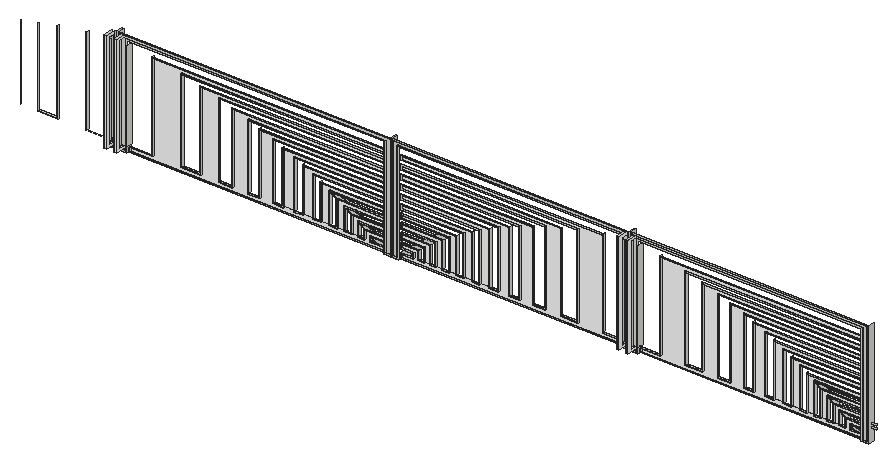
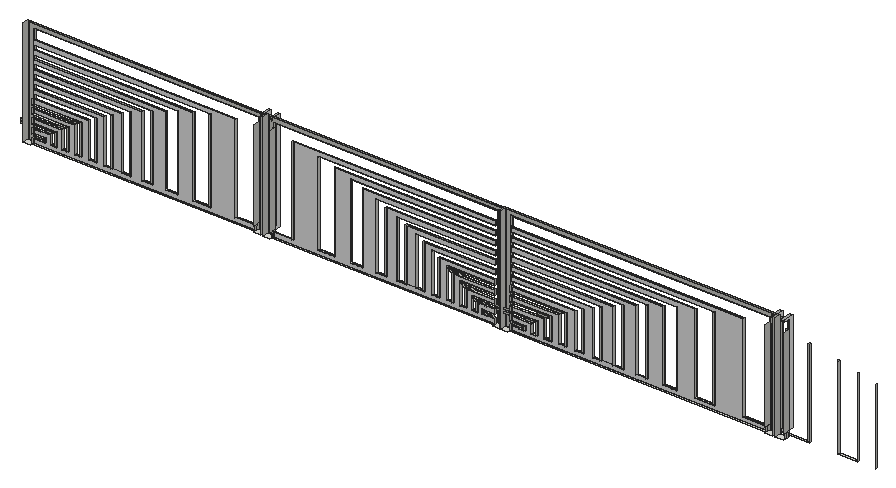
# SketchUp Ruby script. Lengths in inches.
U = 1.inch
M = Sketchup.active_model
def pt(a) = Geom::Point3d.new(a.map { |v| v * U })
def face(e, loops, mat)
  f = e.add_face(loops[0].map { |a| pt(a) })
  loops[1..].each { |l| e.add_face(l.map { |a| pt(a) }).erase! }
  f.material = f.back_material = mat if mat
  f
end
# faces: each face lists its corners as indices into pts; further lists are holes
def faces(e, pts, list, mat = nil) = list.each { |f| face(e, (f[0].is_a?(Array) ? f : [f]).map { |l| l.map { |i| pts[i] } }, mat) }
# xy, xz, yz: faces in a plane at the given z, y or x. An outline is a flat list of corners, or four numbers for a rectangle; further outlines are holes
def ring(l) = l.size == 4 ? [[l[0], l[1]], [l[2], l[1]], [l[2], l[3]], [l[0], l[3]]] : l.each_slice(2).to_a
def flat(e, list, mat, &to3) = list.each { |f| face(e, (f[0].is_a?(Array) ? f : [f]).map { |l| ring(l).map { |u, v| to3.(u, v) } }, mat) }
def xy(e, z, list, mat = nil) = flat(e, list, mat) { |x, y| [x, y, z] }
def xz(e, y, list, mat = nil) = flat(e, list, mat) { |x, z| [x, y, z] }
def yz(e, x, list, mat = nil) = flat(e, list, mat) { |y, z| [x, y, z] }
def lines(e, pts, list) = list.each { |a, b| e.add_line(pt(pts[a]), pt(pts[b])) }
# prism: a flat outline (further loops are holes) pulled along v
def prism(e, loops, v, mat = nil)
  f = face(e, loops, mat); d = Geom::Vector3d.new(v.map { |x| x * U })
  f.pushpull(f.normal.samedirection?(d) ? d.length : -d.length)
end
def box(e, o, s, mat = nil) = prism(e, [[o, [o[0] + s[0], o[1], o[2]], [o[0] + s[0], o[1] + s[1], o[2]], [o[0], o[1] + s[1], o[2]]]], [0, 0, s[2]], mat)
def at(x, y, z, deg = 0) = Geom::Transformation.translation(pt([x, y, z])) * Geom::Transformation.rotation(ORIGIN, Z_AXIS, deg.degrees)
def axes(o, x, y, z) = Geom::Transformation.new([*x, 0, *y, 0, *z, 0, *pt(o).to_a, 1])
def part(name) = M.definitions.add(name)
# library, detail: a bought-in or finely detailed component or shape, given as its bounding box
def library(name, o, s) = part(name).tap { |d| box(d.entities, o, s) }
def detail(e, o, s) = box(e.add_group.entities, o, s)
def put(e, d, t, mat = nil) = e.add_instance(d, t).tap { |i| i.material = mat if mat }
def group(e, t, mat = nil) = e.add_group.tap { |g| g.transformation = t; g.material = mat if mat }.entities
root = M.entities
M.materials.add("[Color_000]").color = [255, 255, 255]
xy(root,0,[[821.45,11.31,827.35,15.56],[828.58,11.31,834.47,15.56],[1013.27,11.31,1019.16,15.56],[1018.58,11.31,1023.71,15.56],[1179.26,11.31,1184.39,15.56],
  [1185.46,11.31,1190.59,15.56],[1346.14,11.31,1351.27,15.56],[834.47,12.93,1013.27,14.31],[1023.71,12.93,1179.26,14.31],[1190.59,12.93,1346.14,14.31]])
xy(root,0.49,[[835.26,12.93,1012.48,13.56],[1024.39,12.93,1178.58,13.56],[1191.27,12.93,1345.46,13.56]])
xy(root,0.7,[[822.57,11.31,826.23,11.81],[829.7,11.31,833.35,11.81],[1014.39,11.31,1018.04,11.81],[1019.55,11.31,1022.73,11.81],[1180.23,11.31,1183.41,11.81],
  [1186.43,11.31,1189.61,11.81],[1347.11,11.31,1350.3,11.81]])
xy(root,2.12,[[823.54,4.75,825.37,11.81],[830.56,4.75,832.38,11.81],[1181.08,4.75,1182.66,11.81],[1187.18,4.75,1188.77,11.81]],"[Color_000]")
xy(root,3.2,[[771.16,12.93,785.19,13.56],[804.64,12.93,820.67,13.56],[835.26,12.93,851.28,13.56],[870.74,12.93,884.76,13.56],[897.07,12.93,907.12,13.56],
  [917.52,12.93,926.1,13.56],[934.55,12.93,942.21,13.56],[949.3125,12.93,956.23,13.56],[962.35,12.93,968.64,13.56],[974.05,12.93,979.79,13.56],
  [984.5625,12.93,989.91,13.56],[993.96,12.93,999.18,13.56],[1002.58,12.93,1006.64,13.56],[1006.64,12.93,1012.48,13.56],[1024.39,12.93,1029.48,13.56],
  [1029.48,12.93,1033,13.56],[1035.96,12.93,1040.51,13.56],[1044.03,12.93,1048.68,13.56],[1052.83,12.93,1057.83,13.56],[1062.53,12.93,1068,13.56],
  [1073.33,12.93,1079.35,13.56],[1085.53,12.93,1092.19,13.56],[1099.55,12.93,1107,13.56],[1116.06,12.93,1124.8,13.56],[1135.51,12.93,1147.71,13.56],
  [1164.63,12.93,1178.58,13.56],[1191.27,12.93,1205.21,13.56],[1222.14,12.93,1234.34,13.56],[1245.05,12.93,1253.79,13.56],[1262.84,12.93,1270.3,13.56],
  [1277.65,12.93,1284.32,13.56],[1290.5,12.93,1296.52,13.56],[1301.84,12.93,1307.3125,13.56],[1312.02,12.93,1317.01,13.56],[1321.17,12.93,1325.82,13.56],
  [1329.34,12.93,1333.88,13.56],[1336.84,12.93,1340.37,13.56],[1340.37,12.93,1345.46,13.56]])
xy(root,3.52,[[823.54,7.12,825.37,11.81],[830.56,7.12,832.38,11.81],[1181.08,7.12,1182.66,11.81],[1187.18,7.12,1188.77,11.81]],"[Color_000]")
xy(root,3.7,[[771.95,12.93,784.4,12.93,784.4,14.31,771.95,14.17],[871.53,12.93,871.53,14.31,883.97,14.17,883.97,12.93],[897.86,12.93,897.86,14.02,906.33,13.93,906.33,12.93],[918.3125,12.93,918.3125,13.8,925.31,13.73,925.31,12.93],[935.33,12.93,935.33,13.62,941.43,13.55,941.43,12.93],
  [950.1,12.93,950.1,13.46,955.44,13.4,955.44,12.93],[963.14,12.93,963.14,13.32,967.85,13.27,967.85,12.93],[974.83,12.93,974.83,13.19,979,13.15,979,12.93],[985.35,12.93,985.35,13.08,989.12,13.04,989.12,12.93],[994.75,12.93,994.75,12.97,998.39,12.93],
  [998.39,12.93,994.75,12.97,994.75,14.31,998.39,14.31],[1003.37,12.93,1006.64,14.31],[1029.48,12.93,1032.32,14.31],[1036.65,12.93,1039.82,12.93,1039.82,12.97],[1036.65,12.93,1039.82,12.97,1039.82,14.31,1036.65,14.31],
  [1044.71,12.93,1047.99,12.93,1047.99,13.08,1044.71,13.04],[1053.52,12.93,1057.15,12.93,1057.15,13.19,1053.52,13.15],[1063.22,12.93,1067.32,12.93,1067.32,13.32,1063.22,13.27],[1074.02,12.93,1078.67,12.93,1078.67,13.46,1074.02,13.4],[1086.21,12.93,1091.51,12.93,1091.51,13.62,1086.21,13.55],
  [1100.23,12.93,1106.32,12.93,1106.32,13.8,1100.23,13.73],[1116.74,12.93,1124.11,12.93,1124.11,14.02,1116.74,13.93],[1136.19,12.93,1147.02,12.93,1147.02,14.31,1136.19,14.17],[1222.82,12.93,1222.82,14.31,1233.65,14.17,1233.65,12.93],[1245.73,12.93,1245.73,14.02,1253.1,13.93,1253.1,12.93],
  [1263.53,12.93,1263.53,13.8,1269.61,13.73,1269.61,12.93],[1278.34,12.93,1278.34,13.62,1283.64,13.55,1283.64,12.93],[1291.18,12.93,1291.18,13.46,1295.83,13.4,1295.83,12.93],[1302.53,12.93,1302.53,13.32,1306.63,13.27,1306.63,12.93],[1312.7,12.93,1312.7,13.19,1316.33,13.15,1316.33,12.93],
  [1321.85,12.93,1321.85,13.08,1325.13,13.04,1325.13,12.93],[1330.03,12.93,1330.03,12.97,1333.2,12.93],[1333.2,12.93,1330.03,12.97,1330.03,14.31,1333.2,14.31],[1337.53,12.93,1340.37,14.31]])
xy(root,6.12,[[1003.37,12.93,1010.01,14.31],[1026.55,12.93,1032.32,14.31],[1337.53,12.93,1343.3,14.31]])
xy(root,6.62,[[1002.58,12.93,1010.01,13.56],[1010.01,12.93,1012.48,13.56],[1024.39,12.93,1026.55,13.56],[1026.55,12.93,1033,13.56],[1336.84,12.93,1343.3,13.56],
  [1343.3,12.93,1345.46,13.56]])
xy(root,9.32,[[999.18,12.93,1005.03,13.56],[1005.03,12.93,1006.64,13.56],[1006.64,12.93,1012.48,13.56],[1024.39,12.93,1029.48,13.56],[1029.48,12.93,1030.875,13.56],
  [1030.875,12.93,1035.96,13.56],[1333.88,12.93,1338.97,13.56],[1338.97,12.93,1340.37,13.56],[1340.37,12.93,1345.46,13.56]])
xy(root,9.82,[[998.39,12.93,1005.03,14.31],[1005.03,12.93,1006.64,14.31],[1006.64,12.93,1013.27,14.31],[1023.71,12.93,1029.48,14.31],[1029.48,12.93,1030.875,14.31],
  [1030.875,12.93,1036.65,14.31],[1333.2,12.93,1338.97,14.31],[1338.97,12.93,1340.37,14.31],[1340.37,12.93,1346.14,14.31]])
xy(root,12.24,[[994.75,12.93,1001.75,14.31],[1001.75,12.93,1013.27,14.31],[1023.71,12.93,1033.73,14.31],[1033.73,12.93,1039.82,14.31],[1330.03,12.93,1336.12,14.31],
  [1336.12,12.93,1346.14,14.31]])
xy(root,12.74,[[993.96,12.93,1001.75,13.56],[1001.75,12.93,1012.48,13.56],[1024.39,12.93,1033.73,13.56],[1033.73,12.93,1040.51,13.56],[1329.34,12.93,1336.12,13.56],
  [1336.12,12.93,1345.46,13.56]])
xy(root,15.44,[[989.91,12.93,996.13,13.56],[996.13,12.93,1012.48,13.56],[1024.39,12.93,1038.62,13.56],[1038.62,12.93,1044.03,13.56],[1325.82,12.93,1331.23,13.56],
  [1331.23,12.93,1345.46,13.56]])
xy(root,15.9375,[[989.12,12.93,996.13,14.31],[996.13,12.93,1013.27,14.31],[1023.71,12.93,1038.62,14.31],[1038.62,12.93,1044.71,14.31],[1325.13,12.93,1331.23,14.31],
  [1331.23,12.93,1346.14,14.31]])
xy(root,18.36,[[985.35,12.93,992.44,14.31],[992.44,12.93,1013.27,14.31],[1023.71,12.93,1041.83,14.31],[1041.83,12.93,1047.99,14.31],[1321.85,12.93,1328.02,14.31],
  [1328.02,12.93,1346.14,14.31]])
xy(root,18.86,[[984.5625,12.93,992.44,13.56],[992.44,12.93,1012.48,13.56],[1024.39,12.93,1041.83,13.56],[1041.83,12.93,1048.68,13.56],[1321.17,12.93,1328.02,13.56],
  [1328.02,12.93,1345.46,13.56]])
xy(root,21.57,[[979.79,12.93,986.45,13.56],[986.45,12.93,1012.48,13.56],[1024.39,12.93,1047.04,13.56],[1047.04,12.93,1052.83,13.56],[1317.01,12.93,1322.8125,13.56],
  [1322.8125,12.93,1345.46,13.56]])
xy(root,22.06,[[979,12.93,986.45,14.31],[986.45,12.93,1013.27,14.31],[1023.71,12.93,1047.04,14.31],[1047.04,12.93,1053.52,14.31],[1316.33,12.93,1322.8125,14.31],
  [1322.8125,12.93,1346.14,14.31]])
xy(root,24.48,[[974.83,12.93,982.29,14.31],[982.29,12.93,1013.27,14.31],[1023.71,12.93,1050.66,14.31],[1050.66,12.93,1057.15,14.31],[1312.7,12.93,1319.1875,14.31],
  [1319.1875,12.93,1346.14,14.31]])
xy(root,24.98,[[974.05,12.93,982.29,13.56],[982.29,12.93,1012.48,13.56],[1024.39,12.93,1050.66,13.56],[1050.66,12.93,1057.83,13.56],[1312.02,12.93,1319.1875,13.56],
  [1319.1875,12.93,1345.46,13.56]])
xz(root,4.75,[[823.54,2.12,825.37,72.7],[830.56,2.12,832.38,72.7],[1181.08,2.12,1182.66,72.7],[1187.18,2.12,1188.77,72.7]],"[Color_000]")
xz(root,7.12,[[823.54,3.52,825.37,71.3],[830.56,3.52,832.38,71.3],[1181.08,3.52,1182.66,71.3],[1187.18,3.52,1188.77,71.3]],"[Color_000]")
xz(root,11.31,[[[828.58,0,828.58,73.9,1019.16,73.9,1019.16,0,1013.27,0,1013.27,70.2,834.47,70.2,834.47,0],[829.7,0.7,833.35,0.7,833.35,70.9,1014.39,70.9,1014.39,0.7,1018.04,0.7,1018.04,73.2,829.7,73.2]],[[1018.58,0,1023.71,0,1023.71,70.2,1179.26,70.2,1179.26,0,1184.39,0,1184.39,73.9,1018.58,73.9],[1019.55,0.7,1019.55,73.2,1183.41,73.2,1183.41,0.7,1180.23,0.7,1180.23,70.9,1022.73,70.9,1022.73,0.7]],[[1185.46,0,1185.46,73.9,1351.27,73.9,1351.27,0,1346.14,0,1346.14,70.2,1190.59,70.2,1190.59,0],[1186.43,0.7,1189.61,0.7,1189.61,70.9,1347.11,70.9,1347.11,0.7,1350.3,0.7,1350.3,73.2,1186.43,73.2]]])
xz(root,11.81,[[[829.7,0.7,829.7,73.2,1018.04,73.2,1018.04,0.7,1014.39,0.7,1014.39,70.9,833.35,70.9,833.35,0.7],[830.56,71.3,832.38,72.7],[830.56,2.12,832.38,3.52]],[[1019.55,0.7,1022.73,0.7,1022.73,70.9,1180.23,70.9,1180.23,0.7,1183.41,0.7,1183.41,73.2,1019.55,73.2],[1181.08,71.3,1182.66,72.7],[1181.08,2.12,1182.66,3.52]],[[1186.43,0.7,1186.43,73.2,1350.3,73.2,1350.3,0.7,1347.11,0.7,1347.11,70.9,1189.61,70.9,1189.61,0.7],[1187.18,71.3,1188.77,72.7],[1187.18,2.12,1188.77,3.52]]])
xz(root,12.93,[[[834.47,0,834.47,3.7,850.5,3.7,850.5,64.91,1013.27,64.91,1013.27,61.21,871.53,61.21,871.53,3.7,883.97,3.7,883.97,58.79,1013.27,58.79,1013.27,55.09,897.86,55.09,897.86,3.7,906.33,3.7,906.33,52.67,1013.27,52.67,1013.27,48.97,918.3125,48.97,918.3125,3.7,925.31,3.7,925.31,46.54,1013.27,46.54,1013.27,42.85,935.33,42.85,935.33,3.7,941.43,3.7,941.43,40.42,1013.27,40.42,1013.27,36.73,950.1,36.73,950.1,3.7,955.44,3.7,955.44,34.3,1013.27,34.3,1013.27,30.61,963.14,30.61,963.14,3.7,967.85,3.7,967.85,28.18,1013.27,28.18,1013.27,24.48,974.83,24.48,974.83,3.7,979,3.7,979,22.06,1013.27,22.06,1013.27,18.36,985.35,18.36,985.35,3.7,989.12,3.7,989.12,15.9375,1013.27,15.9375,1013.27,12.24,994.75,12.24,994.75,3.7,998.39,3.7,998.39,9.82,1013.27,9.82,1013.27,6.12,1003.37,6.12,1003.37,3.7,1013.27,3.7,1013.27,0],[835.26,0.49,1012.48,0.49,1012.48,3.2,1002.58,3.2,1002.58,6.62,1012.48,6.62,1012.48,9.32,999.18,9.32,999.18,3.2,993.96,3.2,993.96,12.74,1012.48,12.74,1012.48,15.44,989.91,15.44,989.91,3.2,984.5625,3.2,984.5625,18.86,1012.48,18.86,1012.48,21.57,979.79,21.57,979.79,3.2,974.05,3.2,974.05,24.98,1012.48,24.98,1012.48,27.6875,968.64,27.6875,968.64,3.2,962.35,3.2,962.35,31.1,1012.48,31.1,1012.48,33.81,956.23,33.81,956.23,3.2,949.3125,3.2,949.3125,37.22,1012.48,37.22,1012.48,39.93,942.21,39.93,942.21,3.2,934.55,3.2,934.55,43.34,1012.48,43.34,1012.48,46.05,926.1,46.05,926.1,3.2,917.52,3.2,917.52,49.46,1012.48,49.46,1012.48,52.17,907.12,52.17,907.12,3.2,897.07,3.2,897.07,55.59,1012.48,55.59,1012.48,58.29,884.76,58.29,884.76,3.2,870.74,3.2,870.74,61.71,1012.48,61.71,1012.48,64.41,851.28,64.41,851.28,3.2,835.26,3.2]],[[1023.71,0,1179.26,0,1179.26,3.7,1165.32,3.7,1165.32,64.91,1023.71,64.91,1023.71,61.21,1147.02,61.21,1147.02,3.7,1136.19,3.7,1136.19,58.79,1023.71,58.79,1023.71,55.09,1124.11,55.09,1124.11,3.7,1116.74,3.7,1116.74,52.67,1023.71,52.67,1023.71,48.97,1106.32,48.97,1106.32,3.7,1100.23,3.7,1100.23,46.54,1023.71,46.54,1023.71,42.85,1091.51,42.85,1091.51,3.7,1086.21,3.7,1086.21,40.42,1023.71,40.42,1023.71,36.73,1078.67,36.73,1078.67,3.7,1074.02,3.7,1074.02,34.3,1023.71,34.3,1023.71,30.61,1067.32,30.61,1067.32,3.7,1063.22,3.7,1063.22,28.18,1023.71,28.18,1023.71,24.48,1057.15,24.48,1057.15,3.7,1053.52,3.7,1053.52,22.06,1023.71,22.06,1023.71,18.36,1047.99,18.36,1047.99,3.7,1044.71,3.7,1044.71,15.9375,1023.71,15.9375,1023.71,12.24,1039.82,12.24,1039.82,3.7,1036.65,3.7,1036.65,9.82,1023.71,9.82,1023.71,6.12,1032.32,6.12,1032.32,3.7,1023.71,3.7],[1024.39,0.49,1024.39,3.2,1033,3.2,1033,6.62,1024.39,6.62,1024.39,9.32,1035.96,9.32,1035.96,3.2,1040.51,3.2,1040.51,12.74,1024.39,12.74,1024.39,15.44,1044.03,15.44,1044.03,3.2,1048.68,3.2,1048.68,18.86,1024.39,18.86,1024.39,21.57,1052.83,21.57,1052.83,3.2,1057.83,3.2,1057.83,24.98,1024.39,24.98,1024.39,27.6875,1062.53,27.6875,1062.53,3.2,1068,3.2,1068,31.1,1024.39,31.1,1024.39,33.81,1073.33,33.81,1073.33,3.2,1079.35,3.2,1079.35,37.22,1024.39,37.22,1024.39,39.93,1085.53,39.93,1085.53,3.2,1092.19,3.2,1092.19,43.34,1024.39,43.34,1024.39,46.05,1099.55,46.05,1099.55,3.2,1107,3.2,1107,49.46,1024.39,49.46,1024.39,52.17,1116.06,52.17,1116.06,3.2,1124.8,3.2,1124.8,55.59,1024.39,55.59,1024.39,58.29,1135.51,58.29,1135.51,3.2,1147.71,3.2,1147.71,61.71,1024.39,61.71,1024.39,64.41,1164.63,64.41,1164.63,3.2,1178.58,3.2,1178.58,0.49]],[[1190.59,0,1190.59,3.7,1204.53,3.7,1204.53,64.91,1346.14,64.91,1346.14,61.21,1222.82,61.21,1222.82,3.7,1233.65,3.7,1233.65,58.79,1346.14,58.79,1346.14,55.09,1245.73,55.09,1245.73,3.7,1253.1,3.7,1253.1,52.67,1346.14,52.67,1346.14,48.97,1263.53,48.97,1263.53,3.7,1269.61,3.7,1269.61,46.54,1346.14,46.54,1346.14,42.85,1278.34,42.85,1278.34,3.7,1283.64,3.7,1283.64,40.42,1346.14,40.42,1346.14,36.73,1291.18,36.73,1291.18,3.7,1295.83,3.7,1295.83,34.3,1346.14,34.3,1346.14,30.61,1302.53,30.61,1302.53,3.7,1306.63,3.7,1306.63,28.18,1346.14,28.18,1346.14,24.48,1312.7,24.48,1312.7,3.7,1316.33,3.7,1316.33,22.06,1346.14,22.06,1346.14,18.36,1321.85,18.36,1321.85,3.7,1325.13,3.7,1325.13,15.9375,1346.14,15.9375,1346.14,12.24,1330.03,12.24,1330.03,3.7,1333.2,3.7,1333.2,9.82,1346.14,9.82,1346.14,6.12,1337.53,6.12,1337.53,3.7,1346.14,3.7,1346.14,0],[1191.27,0.49,1345.46,0.49,1345.46,3.2,1336.84,3.2,1336.84,6.62,1345.46,6.62,1345.46,9.32,1333.88,9.32,1333.88,3.2,1329.34,3.2,1329.34,12.74,1345.46,12.74,1345.46,15.44,1325.82,15.44,1325.82,3.2,1321.17,3.2,1321.17,18.86,1345.46,18.86,1345.46,21.57,1317.01,21.57,1317.01,3.2,1312.02,3.2,1312.02,24.98,1345.46,24.98,1345.46,27.6875,1307.3125,27.6875,1307.3125,3.2,1301.84,3.2,1301.84,31.1,1345.46,31.1,1345.46,33.81,1296.52,33.81,1296.52,3.2,1290.5,3.2,1290.5,37.22,1345.46,37.22,1345.46,39.93,1284.32,39.93,1284.32,3.2,1277.65,3.2,1277.65,43.34,1345.46,43.34,1345.46,46.05,1270.3,46.05,1270.3,3.2,1262.84,3.2,1262.84,49.46,1345.46,49.46,1345.46,52.17,1253.79,52.17,1253.79,3.2,1245.05,3.2,1245.05,55.59,1345.46,55.59,1345.46,58.29,1234.34,58.29,1234.34,3.2,1222.14,3.2,1222.14,61.71,1345.46,61.71,1345.46,64.41,1205.21,64.41,1205.21,3.2,1191.27,3.2]],[1006.64,3.7,1003.37,6.12,1010.01,6.12,1013.27,3.7],[1023.71,3.7,1029.48,3.7,1032.32,6.12,1026.55,6.12],
  [1340.37,3.7,1337.53,6.12,1343.3,6.12,1346.14,3.7],[998.39,9.82,998.07,10.06,994.75,12.24,1001.75,12.24,1001.84,12.18,1005.03,9.82],[1030.875,9.82,1036.65,9.82,1036.93,10.06,1039.82,12.24,1033.73,12.24,1033.65,12.18],[1333.2,9.82,1332.92,10.06,1330.03,12.24,1336.12,12.24,1336.2,12.18,1338.97,9.82],[989.12,15.9375,986.06,17.95,985.35,18.36,992.44,18.36,996.13,15.9375],
  [1038.62,15.9375,1044.71,15.9375,1047.38,17.95,1047.99,18.36,1041.83,18.36],[1325.13,15.9375,1322.46,17.95,1321.85,18.36,1328.02,18.36,1331.23,15.9375],[979,22.06,974.83,24.48,982.29,24.48,986.45,22.06],[1047.04,22.06,1053.52,22.06,1057.15,24.48,1050.66,24.48],[1316.33,22.06,1312.7,24.48,1319.1875,24.48,1322.8125,22.06]])
xz(root,13.24,[[1014.6875,9.21,1018.58,10.5],[1019.16,9.21,1023.63,10.5],[1351.27,9.21,1355.16,10.5],[1014.6875,11.42,1018.58,12.71],[1019.16,11.42,1023.63,12.71],
  [1351.27,11.42,1355.16,12.71]])
xz(root,13.56,[[835.26,0.49,835.26,3.2,851.28,3.2,851.28,64.41,1012.48,64.41,1012.48,61.71,870.74,61.71,870.74,3.2,884.76,3.2,884.76,58.29,1012.48,58.29,1012.48,55.59,897.07,55.59,897.07,3.2,907.12,3.2,907.12,52.17,1012.48,52.17,1012.48,49.46,917.52,49.46,917.52,3.2,926.1,3.2,926.1,46.05,1012.48,46.05,1012.48,43.34,934.55,43.34,934.55,3.2,942.21,3.2,942.21,39.93,1012.48,39.93,1012.48,37.22,949.3125,37.22,949.3125,3.2,956.23,3.2,956.23,33.81,1012.48,33.81,1012.48,31.1,962.35,31.1,962.35,3.2,968.64,3.2,968.64,27.6875,1012.48,27.6875,1012.48,24.98,974.05,24.98,974.05,3.2,979.79,3.2,979.79,21.57,1012.48,21.57,1012.48,18.86,984.5625,18.86,984.5625,3.2,989.91,3.2,989.91,15.44,1012.48,15.44,1012.48,12.74,993.96,12.74,993.96,3.2,999.18,3.2,999.18,9.32,1012.48,9.32,1012.48,6.62,1002.58,6.62,1002.58,3.2,1012.48,3.2,1012.48,0.49],[1024.39,0.49,1178.58,0.49,1178.58,3.2,1164.63,3.2,1164.63,64.41,1024.39,64.41,1024.39,61.71,1147.71,61.71,1147.71,3.2,1135.51,3.2,1135.51,58.29,1024.39,58.29,1024.39,55.59,1124.8,55.59,1124.8,3.2,1116.06,3.2,1116.06,52.17,1024.39,52.17,1024.39,49.46,1107,49.46,1107,3.2,1099.55,3.2,1099.55,46.05,1024.39,46.05,1024.39,43.34,1092.19,43.34,1092.19,3.2,1085.53,3.2,1085.53,39.93,1024.39,39.93,1024.39,37.22,1079.35,37.22,1079.35,3.2,1073.33,3.2,1073.33,33.81,1024.39,33.81,1024.39,31.1,1068,31.1,1068,3.2,1062.53,3.2,1062.53,27.6875,1024.39,27.6875,1024.39,24.98,1057.83,24.98,1057.83,3.2,1052.83,3.2,1052.83,21.57,1024.39,21.57,1024.39,18.86,1048.68,18.86,1048.68,3.2,1044.03,3.2,1044.03,15.44,1024.39,15.44,1024.39,12.74,1040.51,12.74,1040.51,3.2,1035.96,3.2,1035.96,9.32,1024.39,9.32,1024.39,6.62,1033,6.62,1033,3.2,1024.39,3.2],[1191.27,0.49,1191.27,3.2,1205.21,3.2,1205.21,64.41,1345.46,64.41,1345.46,61.71,1222.14,61.71,1222.14,3.2,1234.34,3.2,1234.34,58.29,1345.46,58.29,1345.46,55.59,1245.05,55.59,1245.05,3.2,1253.79,3.2,1253.79,52.17,1345.46,52.17,1345.46,49.46,1262.84,49.46,1262.84,3.2,1270.3,3.2,1270.3,46.05,1345.46,46.05,1345.46,43.34,1277.65,43.34,1277.65,3.2,1284.32,3.2,1284.32,39.93,1345.46,39.93,1345.46,37.22,1290.5,37.22,1290.5,3.2,1296.52,3.2,1296.52,33.81,1345.46,33.81,1345.46,31.1,1301.84,31.1,1301.84,3.2,1307.3125,3.2,1307.3125,27.6875,1345.46,27.6875,1345.46,24.98,1312.02,24.98,1312.02,3.2,1317.01,3.2,1317.01,21.57,1345.46,21.57,1345.46,18.86,1321.17,18.86,1321.17,3.2,1325.82,3.2,1325.82,15.44,1345.46,15.44,1345.46,12.74,1329.34,12.74,1329.34,3.2,1333.88,3.2,1333.88,9.32,1345.46,9.32,1345.46,6.62,1336.84,6.62,1336.84,3.2,1345.46,3.2,1345.46,0.49]],"[Color_000]")
yz(root,758.85,[[12.93,3.2,13.56,55.59]])
yz(root,771.16,[[12.93,3.2,13.56,58.29]])
yz(root,784.4,[[12.93,3.7,14.31,61.21]])
yz(root,785.19,[[12.93,3.2,13.56,61.71]])
yz(root,804.64,[[12.93,3.2,13.56,64.41]])
yz(root,805.43,[[12.93,3.7,14.31,64.91]])
yz(root,820.67,[[12.93,0.49,13.56,3.2]])
yz(root,821.45,[[11.31,0,12.93,3.7],[12.93,0,14.31,3.7],[11.31,3.7,15.56,66.96]])
yz(root,822.57,[[11.31,0.7,11.81,3.7],[11.31,3.7,11.81,66.96]])
yz(root,823.54,[[4.75,2.12,4.75,72.7,11.81,72.7,11.81,71.3,7.12,71.3,7.12,3.52,11.81,3.52,11.81,2.12]],"[Color_000]")
yz(root,825.37,[[4.75,2.12,11.81,2.12,11.81,3.52,7.12,3.52,7.12,71.3,11.81,71.3,11.81,72.7,4.75,72.7]],"[Color_000]")
yz(root,826.23,[[11.31,0.7,11.81,73.2]])
yz(root,827.35,[[11.31,0,15.56,73.9]])
yz(root,828.58,[[11.31,0,15.56,73.9]])
yz(root,829.7,[[11.31,0.7,11.81,73.2]])
yz(root,830.56,[[4.75,2.12,11.81,2.12,11.81,3.52,7.12,3.52,7.12,71.3,11.81,71.3,11.81,72.7,4.75,72.7]],"[Color_000]")
yz(root,832.38,[[4.75,2.12,4.75,72.7,11.81,72.7,11.81,71.3,7.12,71.3,7.12,3.52,11.81,3.52,11.81,2.12]],"[Color_000]")
yz(root,833.35,[[11.31,0.7,11.81,3.7],[11.31,3.7,11.81,66.96]])
yz(root,834.47,[[11.31,0,12.93,3.7],[12.93,0,14.31,3.7],[11.31,3.7,15.56,66.96]])
yz(root,835.26,[[12.93,0.49,13.56,3.2]])
yz(root,850.5,[[12.93,3.7,14.31,64.91]])
yz(root,851.28,[[12.93,3.2,13.56,64.41]])
yz(root,870.74,[[12.93,3.2,13.56,61.71]])
yz(root,871.53,[[12.93,3.7,14.31,61.21]])
yz(root,884.76,[[12.93,3.2,13.56,58.29]])
yz(root,897.07,[[12.93,3.2,13.56,55.59]])
yz(root,907.12,[[12.93,3.2,13.56,52.17]])
yz(root,917.52,[[12.93,3.2,13.56,49.46]])
yz(root,918.3125,[[12.93,3.7,14.31,48.97]])
yz(root,925.31,[[12.93,3.7,14.31,46.54]])
yz(root,926.1,[[12.93,3.2,13.56,46.05]])
yz(root,934.55,[[12.93,3.2,13.56,43.34]])
yz(root,935.33,[[12.93,3.7,14.31,42.85]])
yz(root,941.43,[[12.93,3.7,14.31,40.42]])
yz(root,942.21,[[12.93,3.2,13.56,39.93]])
yz(root,949.3125,[[12.93,3.2,13.56,37.22]])
yz(root,950.1,[[12.93,3.7,14.31,36.73]])
yz(root,955.44,[[12.93,3.7,14.31,34.3]])
yz(root,956.23,[[12.93,3.2,13.56,33.81]])
yz(root,962.35,[[12.93,3.2,13.56,31.1]])
yz(root,963.14,[[12.93,3.7,14.31,30.61]])
yz(root,967.85,[[12.93,3.7,14.31,28.18]])
yz(root,968.64,[[12.93,3.2,13.56,27.6875]])
yz(root,974.05,[[12.93,3.2,13.56,24.98]])
yz(root,974.83,[[12.93,3.7,14.31,24.48]])
yz(root,979,[[12.93,3.7,14.31,22.06]])
yz(root,979.79,[[12.93,3.2,13.56,21.57]])
yz(root,984.5625,[[12.93,3.2,13.56,18.86]])
yz(root,985.35,[[12.93,3.7,14.31,18.36]])
yz(root,989.12,[[12.93,3.7,14.31,15.9375]])
yz(root,989.91,[[12.93,3.2,13.56,15.44]])
yz(root,993.96,[[12.93,3.2,13.56,12.74]])
yz(root,994.75,[[12.93,3.7,14.31,12.24]])
yz(root,998.39,[[12.93,3.7,14.31,9.82]])
yz(root,999.18,[[12.93,3.2,13.56,9.32]])
yz(root,1002.58,[[12.93,3.2,13.56,6.62]])
yz(root,1003.37,[[12.93,3.7,14.31,6.12]])
yz(root,1012.48,[[12.93,0.49,13.56,3.2],[12.93,6.62,13.56,9.32],[12.93,12.74,13.56,15.44],[12.93,18.86,13.56,21.57],[12.93,24.98,13.56,27.6875]])
yz(root,1013.27,[[12.93,0,14.31,3.7],[12.93,6.12,14.31,9.82],[12.93,12.24,14.31,15.9375],[12.93,18.36,14.31,22.06],[12.93,24.48,14.31,28.18]])
yz(root,1014.39,[[11.31,0.7,11.81,70.9]])
yz(root,1018.04,[[11.31,0.7,11.81,73.2]])
yz(root,1018.58,[[[11.31,0,15.56,73.9],[13.24,63.67,14.43,64.96],[13.24,61.46,14.43,62.75],[13.24,11.42,14.43,12.71],[13.24,9.21,14.43,10.5]]])
yz(root,1019.16,[[[11.31,0,15.56,73.9],[13.24,63.67,14.43,64.96],[13.24,61.46,14.43,62.75],[13.24,11.42,14.43,12.71],[13.24,9.21,14.43,10.5]]])
yz(root,1019.55,[[11.31,0.7,11.81,73.2]])
yz(root,1022.73,[[11.31,0.7,11.81,70.9]])
yz(root,1023.71,[[12.93,0,14.31,3.7],[12.93,6.12,14.31,9.82],[12.93,12.24,14.31,15.9375],[12.93,18.36,14.31,22.06],[12.93,24.48,14.31,28.18]])
yz(root,1024.39,[[12.93,0.49,13.56,3.2],[12.93,6.62,13.56,9.32],[12.93,12.74,13.56,15.44],[12.93,18.86,13.56,21.57],[12.93,24.98,13.56,27.6875]])
yz(root,1032.32,[[12.93,3.7,14.31,6.12]])
yz(root,1033,[[12.93,3.2,13.56,6.62]])
yz(root,1035.96,[[12.93,3.2,13.56,9.32]])
yz(root,1036.65,[[12.93,3.7,14.31,9.82]])
yz(root,1039.82,[[12.93,3.7,14.31,12.24]])
yz(root,1040.51,[[12.93,3.2,13.56,12.74]])
yz(root,1044.03,[[12.93,3.2,13.56,15.44]])
yz(root,1044.71,[[12.93,3.7,14.31,15.9375]])
yz(root,1047.99,[[12.93,3.7,14.31,18.36]])
yz(root,1048.68,[[12.93,3.2,13.56,18.86]])
yz(root,1052.83,[[12.93,3.2,13.56,21.57]])
yz(root,1053.52,[[12.93,3.7,14.31,22.06]])
yz(root,1057.15,[[12.93,3.7,14.31,24.48]])
yz(root,1057.83,[[12.93,3.2,13.56,24.98]])
yz(root,1062.53,[[12.93,3.2,13.56,27.6875]])
yz(root,1063.22,[[12.93,3.7,14.31,28.18]])
yz(root,1067.32,[[12.93,3.7,14.31,30.61]])
yz(root,1068,[[12.93,3.2,13.56,31.1]])
yz(root,1073.33,[[12.93,3.2,13.56,33.81]])
yz(root,1074.02,[[12.93,3.7,14.31,34.3]])
yz(root,1078.67,[[12.93,3.7,14.31,36.73]])
yz(root,1079.35,[[12.93,3.2,13.56,37.22]])
yz(root,1085.53,[[12.93,3.2,13.56,39.93]])
yz(root,1086.21,[[12.93,3.7,14.31,40.42]])
yz(root,1091.51,[[12.93,3.7,14.31,42.85]])
yz(root,1092.19,[[12.93,3.2,13.56,43.34]])
yz(root,1099.55,[[12.93,3.2,13.56,46.05]])
yz(root,1100.23,[[12.93,3.7,14.31,46.54]])
yz(root,1106.32,[[12.93,3.7,14.31,48.97]])
yz(root,1107,[[12.93,3.2,13.56,49.46]])
yz(root,1116.06,[[12.93,3.2,13.56,52.17]])
yz(root,1124.8,[[12.93,3.2,13.56,55.59]])
yz(root,1135.51,[[12.93,3.2,13.56,58.29]])
yz(root,1147.02,[[12.93,3.7,14.31,61.21]])
yz(root,1147.71,[[12.93,3.2,13.56,61.71]])
yz(root,1164.63,[[12.93,3.2,13.56,64.41]])
yz(root,1165.32,[[12.93,3.7,14.31,64.91]])
yz(root,1178.58,[[12.93,0.49,13.56,3.2]])
yz(root,1179.26,[[11.31,0,12.93,3.7],[12.93,0,14.31,3.7],[11.31,3.7,15.56,66.96]])
yz(root,1180.23,[[11.31,0.7,11.81,3.7],[11.31,3.7,11.81,66.96]])
yz(root,1181.08,[[4.75,2.12,4.75,72.7,11.81,72.7,11.81,71.3,7.12,71.3,7.12,3.52,11.81,3.52,11.81,2.12]],"[Color_000]")
yz(root,1182.66,[[4.75,2.12,11.81,2.12,11.81,3.52,7.12,3.52,7.12,71.3,11.81,71.3,11.81,72.7,4.75,72.7]],"[Color_000]")
yz(root,1183.41,[[11.31,0.7,11.81,73.2]])
yz(root,1184.39,[[11.31,0,15.56,73.9]])
yz(root,1185.46,[[11.31,0,15.56,73.9]])
yz(root,1186.43,[[11.31,0.7,11.81,73.2]])
yz(root,1187.18,[[4.75,2.12,11.81,2.12,11.81,3.52,7.12,3.52,7.12,71.3,11.81,71.3,11.81,72.7,4.75,72.7]],"[Color_000]")
yz(root,1188.77,[[4.75,2.12,4.75,72.7,11.81,72.7,11.81,71.3,7.12,71.3,7.12,3.52,11.81,3.52,11.81,2.12]],"[Color_000]")
yz(root,1189.61,[[11.31,0.7,11.81,3.7],[11.31,3.7,11.81,66.96]])
yz(root,1190.59,[[11.31,0,12.93,3.7],[12.93,0,14.31,3.7],[11.31,3.7,15.56,66.96]])
yz(root,1191.27,[[12.93,0.49,13.56,3.2]])
yz(root,1204.53,[[12.93,3.7,14.31,64.91]])
yz(root,1205.21,[[12.93,3.2,13.56,64.41]])
yz(root,1222.14,[[12.93,3.2,13.56,61.71]])
yz(root,1222.82,[[12.93,3.7,14.31,61.21]])
yz(root,1234.34,[[12.93,3.2,13.56,58.29]])
yz(root,1245.05,[[12.93,3.2,13.56,55.59]])
yz(root,1253.79,[[12.93,3.2,13.56,52.17]])
yz(root,1262.84,[[12.93,3.2,13.56,49.46]])
yz(root,1263.53,[[12.93,3.7,14.31,48.97]])
yz(root,1269.61,[[12.93,3.7,14.31,46.54]])
yz(root,1270.3,[[12.93,3.2,13.56,46.05]])
yz(root,1277.65,[[12.93,3.2,13.56,43.34]])
yz(root,1278.34,[[12.93,3.7,14.31,42.85]])
yz(root,1283.64,[[12.93,3.7,14.31,40.42]])
yz(root,1284.32,[[12.93,3.2,13.56,39.93]])
yz(root,1290.5,[[12.93,3.2,13.56,37.22]])
yz(root,1291.18,[[12.93,3.7,14.31,36.73]])
yz(root,1295.83,[[12.93,3.7,14.31,34.3]])
yz(root,1296.52,[[12.93,3.2,13.56,33.81]])
yz(root,1301.84,[[12.93,3.2,13.56,31.1]])
yz(root,1302.53,[[12.93,3.7,14.31,30.61]])
yz(root,1306.63,[[12.93,3.7,14.31,28.18]])
yz(root,1307.3125,[[12.93,3.2,13.56,27.6875]])
yz(root,1312.02,[[12.93,3.2,13.56,24.98]])
yz(root,1312.7,[[12.93,3.7,14.31,24.48]])
yz(root,1316.33,[[12.93,3.7,14.31,22.06]])
yz(root,1317.01,[[12.93,3.2,13.56,21.57]])
yz(root,1321.17,[[12.93,3.2,13.56,18.86]])
yz(root,1321.85,[[12.93,3.7,14.31,18.36]])
yz(root,1325.13,[[12.93,3.7,14.31,15.9375]])
yz(root,1325.82,[[12.93,3.2,13.56,15.44]])
yz(root,1329.34,[[12.93,3.2,13.56,12.74]])
yz(root,1330.03,[[12.93,3.7,14.31,12.24]])
yz(root,1333.2,[[12.93,3.7,14.31,9.82]])
yz(root,1333.88,[[12.93,3.2,13.56,9.32]])
yz(root,1336.84,[[12.93,3.2,13.56,6.62]])
yz(root,1337.53,[[12.93,3.7,14.31,6.12]])
yz(root,1345.46,[[12.93,0.49,13.56,3.2],[12.93,6.62,13.56,9.32],[12.93,12.74,13.56,15.44],[12.93,18.86,13.56,21.57],[12.93,24.98,13.56,27.6875]])
yz(root,1346.14,[[12.93,0,14.31,3.7],[12.93,6.12,14.31,9.82],[12.93,12.24,14.31,15.9375],[12.93,18.36,14.31,22.06],[12.93,24.48,14.31,28.18]])
yz(root,1347.11,[[11.31,0.7,11.81,70.9]])
yz(root,1350.3,[[11.31,0.7,11.81,73.2]])
yz(root,1351.27,[[[11.31,0,15.56,73.9],[13.24,63.67,14.43,64.96],[13.24,61.46,14.43,62.75],[13.24,11.42,14.43,12.71],[13.24,9.21,14.43,10.5]]])
p = [[1006.64,14.31,3.7],[1003.37,14.31,6.12],[1003.37,12.93,6.12],[1006.64,12.93,3.7],[1010.01,14.31,6.12],[1013.27,14.31,3.7],
  [1013.27,12.93,3.7],[1010.01,12.93,6.12],[1026.55,14.31,6.12],[1023.71,14.31,3.7],[1023.71,12.93,3.7],[1026.55,12.93,6.12],
  [1029.48,14.31,3.7],[1032.32,14.31,6.12],[1032.32,12.93,6.12],[1029.48,12.93,3.7],[1340.37,14.31,3.7],[1337.53,14.31,6.12],
  [1337.53,12.93,6.12],[1340.37,12.93,3.7],[1343.3,14.31,6.12],[1346.14,14.31,3.7],[1346.14,12.93,3.7],[1343.3,12.93,6.12],
  [998.39,14.31,9.82],[998.07,14.31,10.06],[998.07,12.93,10.06],[998.39,12.93,9.82],[1001.84,14.31,12.18],[1005.03,14.31,9.82],
  [1005.03,12.93,9.82],[1001.84,12.93,12.18],[1033.65,14.31,12.18],[1030.875,14.31,9.82],[1030.875,12.93,9.82],[1033.65,12.93,12.18],
  [1036.65,14.31,9.82],[1036.93,14.31,10.06],[1036.93,12.93,10.06],[1036.65,12.93,9.82],[1333.2,14.31,9.82],[1332.92,14.31,10.06],
  [1332.92,12.93,10.06],[1333.2,12.93,9.82],[1336.2,14.31,12.18],[1338.97,14.31,9.82],[1338.97,12.93,9.82],[1336.2,12.93,12.18],
  [994.75,14.31,12.24],[994.75,12.93,12.24],[1039.82,14.31,12.24],[1039.82,12.93,12.24],[1330.03,14.31,12.24],[1330.03,12.93,12.24],
  [1001.75,14.31,12.24],[1001.75,12.93,12.24],[1033.73,14.31,12.24],[1033.73,12.93,12.24],[1336.12,14.31,12.24],[1336.12,12.93,12.24],
  [989.12,14.31,15.9375],[986.06,14.31,17.95],[986.06,12.93,17.95],[989.12,12.93,15.9375],[992.44,14.31,18.36],[996.13,14.31,15.9375],
  [996.13,12.93,15.9375],[992.44,12.93,18.36],[1041.83,14.31,18.36],[1038.62,14.31,15.9375],[1038.62,12.93,15.9375],[1041.83,12.93,18.36],
  [1044.71,14.31,15.9375],[1047.38,14.31,17.95],[1047.38,12.93,17.95],[1044.71,12.93,15.9375],[1325.13,14.31,15.9375],[1322.46,14.31,17.95],
  [1322.46,12.93,17.95],[1325.13,12.93,15.9375],[1328.02,14.31,18.36],[1331.23,14.31,15.9375],[1331.23,12.93,15.9375],[1328.02,12.93,18.36],
  [985.35,14.31,18.36],[985.35,12.93,18.36],[1047.99,14.31,18.36],[1047.99,12.93,18.36],[1321.85,14.31,18.36],[1321.85,12.93,18.36],
  [979,14.31,22.06],[974.83,14.31,24.48],[974.83,12.93,24.48],[979,12.93,22.06],[982.29,14.31,24.48],[986.45,14.31,22.06],
  [986.45,12.93,22.06],[982.29,12.93,24.48],[1050.66,14.31,24.48],[1047.04,14.31,22.06],[1047.04,12.93,22.06],[1050.66,12.93,24.48],
  [1053.52,14.31,22.06],[1057.15,14.31,24.48],[1057.15,12.93,24.48],[1053.52,12.93,22.06],[1316.33,14.31,22.06],[1312.7,14.31,24.48],
  [1312.7,12.93,24.48],[1316.33,12.93,22.06],[1319.1875,14.31,24.48],[1322.8125,14.31,22.06],[1322.8125,12.93,22.06],[1319.1875,12.93,24.48],
  [967.85,13.27,3.7],[974.83,13.19,3.7],[955.44,13.4,3.7],[963.14,13.32,3.7],[941.43,13.55,3.7],[950.1,13.46,3.7],
  [989.12,13.04,3.7],[994.75,12.97,3.7],[979,13.15,3.7],[985.35,13.08,3.7],[1306.63,13.27,3.7],[1312.7,13.19,3.7],
  [1295.83,13.4,3.7],[1302.53,13.32,3.7],[1283.64,13.55,3.7],[1291.18,13.46,3.7],[1325.13,13.04,3.7],[1330.03,12.97,3.7],
  [1316.33,13.15,3.7],[1321.85,13.08,3.7],[1063.22,13.27,3.7],[1057.15,13.19,3.7],[1074.02,13.4,3.7],[1067.32,13.32,3.7],
  [1086.21,13.55,3.7],[1078.67,13.46,3.7],[1044.71,13.04,3.7],[1039.82,12.97,3.7],[1053.52,13.15,3.7],[1047.99,13.08,3.7]]
faces(root,p,[[0,1,2,3],[4,5,6,7],[8,9,10,11],[12,13,14,15],[16,17,18,19],[20,21,22,23],[24,25,26,27],[28,29,30,31],
  [32,33,34,35],[36,37,38,39],[40,41,42,43],[44,45,46,47],[25,48,49,26],[37,50,51,38],[41,52,53,42],[54,28,31,55],
  [56,32,35,57],[58,44,47,59],[60,61,62,63],[64,65,66,67],[68,69,70,71],[72,73,74,75],[76,77,78,79],[80,81,82,83],
  [61,84,85,62],[73,86,87,74],[77,88,89,78],[90,91,92,93],[94,95,96,97],[98,99,100,101],[102,103,104,105],[106,107,108,109],
  [110,111,112,113]])
lines(root,p,[[114,115],[116,117],[118,119],[120,121],[122,123],[124,125],[126,127],[128,129],[130,131],[132,133],[134,135],[136,137],
  [138,139],[140,141],[142,143]])
